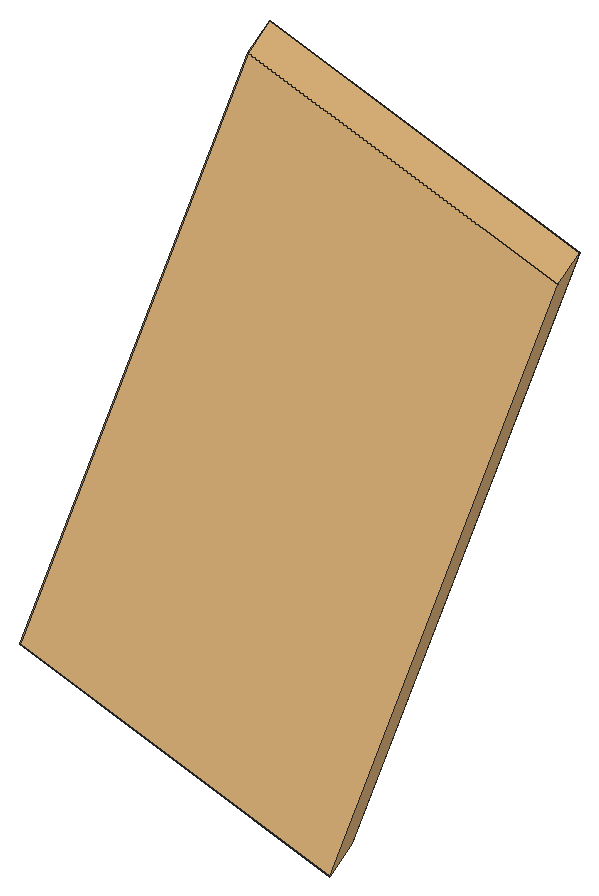
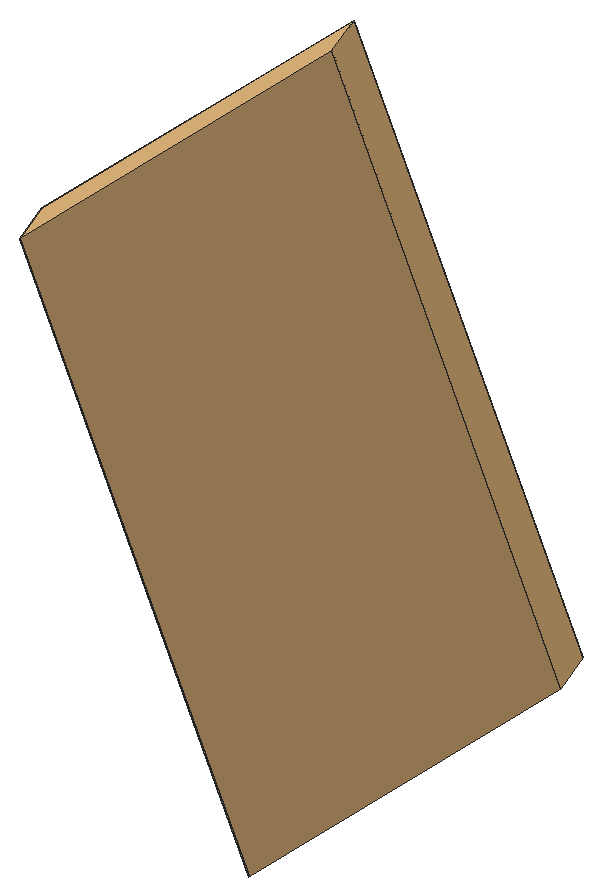
# SketchUp Ruby script. Lengths in inches.
U = 1.inch
M = Sketchup.active_model
def pt(a) = Geom::Point3d.new(a.map { |v| v * U })
def face(e, loops, mat)
  f = e.add_face(loops[0].map { |a| pt(a) })
  loops[1..].each { |l| e.add_face(l.map { |a| pt(a) }).erase! }
  f.material = f.back_material = mat if mat
  f
end
# faces: each face lists its corners as indices into pts; further lists are holes
def faces(e, pts, list, mat = nil) = list.each { |f| face(e, (f[0].is_a?(Array) ? f : [f]).map { |l| l.map { |i| pts[i] } }, mat) }
# xy, xz, yz: faces in a plane at the given z, y or x. An outline is a flat list of corners, or four numbers for a rectangle; further outlines are holes
def ring(l) = l.size == 4 ? [[l[0], l[1]], [l[2], l[1]], [l[2], l[3]], [l[0], l[3]]] : l.each_slice(2).to_a
def flat(e, list, mat, &to3) = list.each { |f| face(e, (f[0].is_a?(Array) ? f : [f]).map { |l| ring(l).map { |u, v| to3.(u, v) } }, mat) }
def xy(e, z, list, mat = nil) = flat(e, list, mat) { |x, y| [x, y, z] }
def xz(e, y, list, mat = nil) = flat(e, list, mat) { |x, z| [x, y, z] }
def yz(e, x, list, mat = nil) = flat(e, list, mat) { |y, z| [x, y, z] }
def lines(e, pts, list) = list.each { |a, b| e.add_line(pt(pts[a]), pt(pts[b])) }
# prism: a flat outline (further loops are holes) pulled along v
def prism(e, loops, v, mat = nil)
  f = face(e, loops, mat); d = Geom::Vector3d.new(v.map { |x| x * U })
  f.pushpull(f.normal.samedirection?(d) ? d.length : -d.length)
end
def box(e, o, s, mat = nil) = prism(e, [[o, [o[0] + s[0], o[1], o[2]], [o[0] + s[0], o[1] + s[1], o[2]], [o[0], o[1] + s[1], o[2]]]], [0, 0, s[2]], mat)
def at(x, y, z, deg = 0) = Geom::Transformation.translation(pt([x, y, z])) * Geom::Transformation.rotation(ORIGIN, Z_AXIS, deg.degrees)
def axes(o, x, y, z) = Geom::Transformation.new([*x, 0, *y, 0, *z, 0, *pt(o).to_a, 1])
def part(name) = M.definitions.add(name)
# library, detail: a bought-in or finely detailed component or shape, given as its bounding box
def library(name, o, s) = part(name).tap { |d| box(d.entities, o, s) }
def detail(e, o, s) = box(e.add_group.entities, o, s)
def put(e, d, t, mat = nil) = e.add_instance(d, t).tap { |i| i.material = mat if mat }
def group(e, t, mat = nil) = e.add_group.tap { |g| g.transformation = t; g.material = mat if mat }.entities
root = M.entities
c1 = library("sm2 st v2 Component\#1",[0,0,0],[29.46,4.93,43.46])
put(root,c1,axes([64.34,87.42,100.43],[0.33346,0.1929,-0.29533],[-0.17149,0.46507,0.0088],[0.17082,0.09033,0.58536]))
